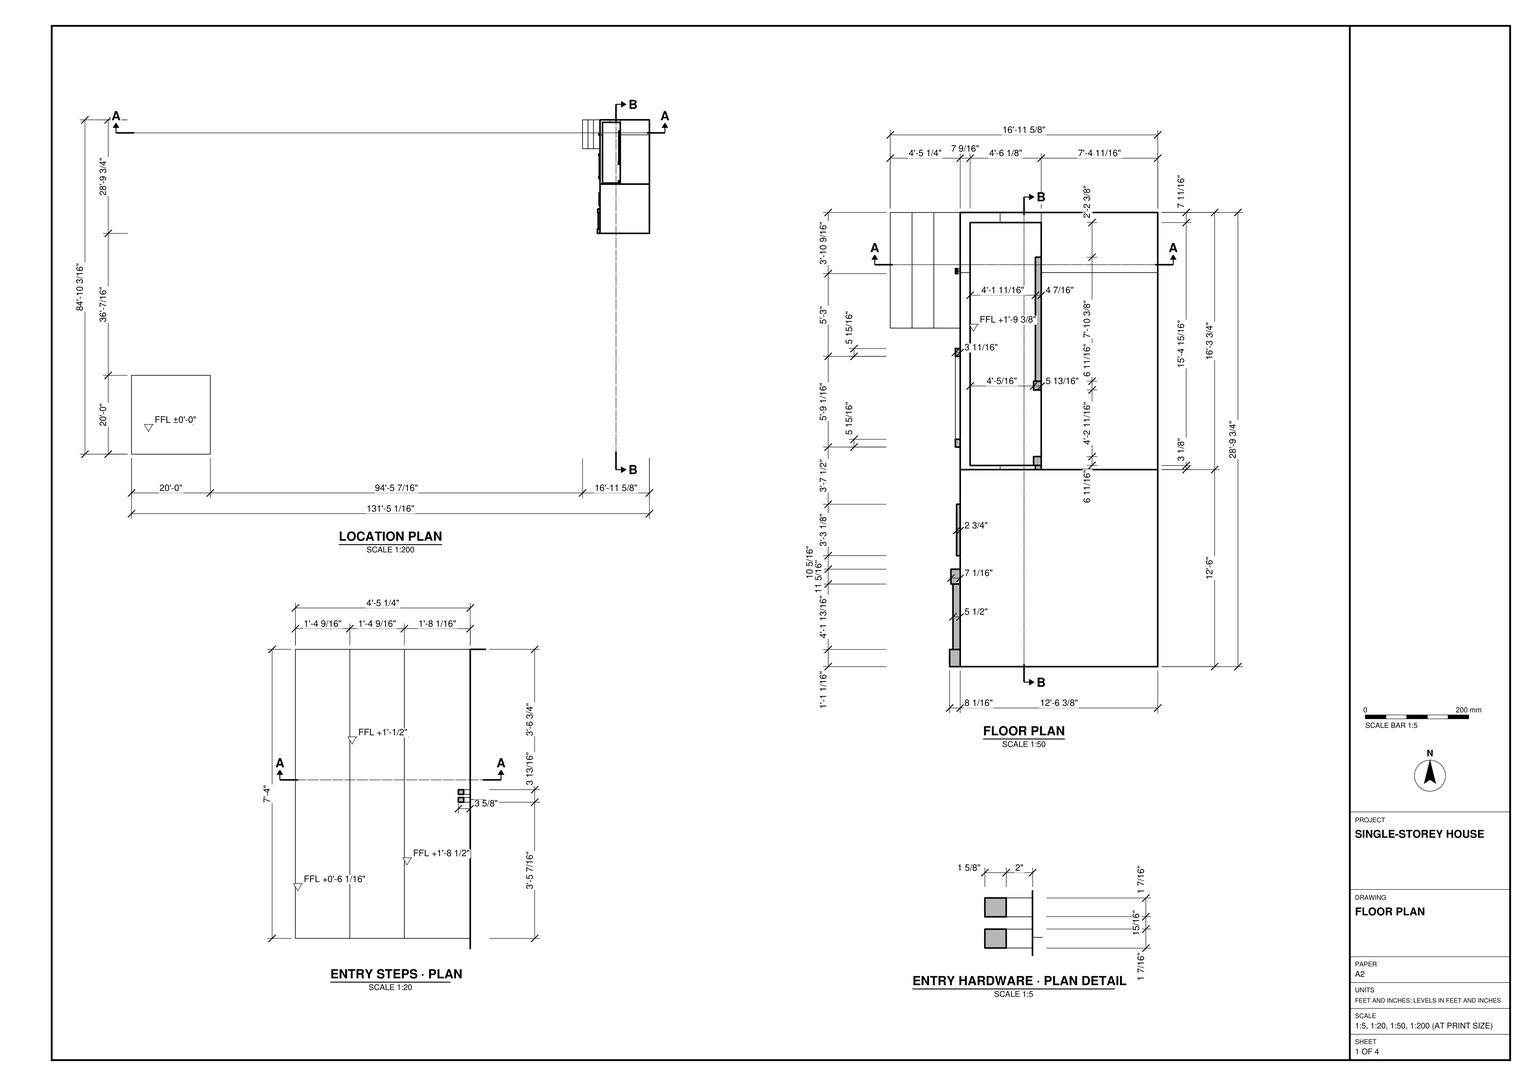
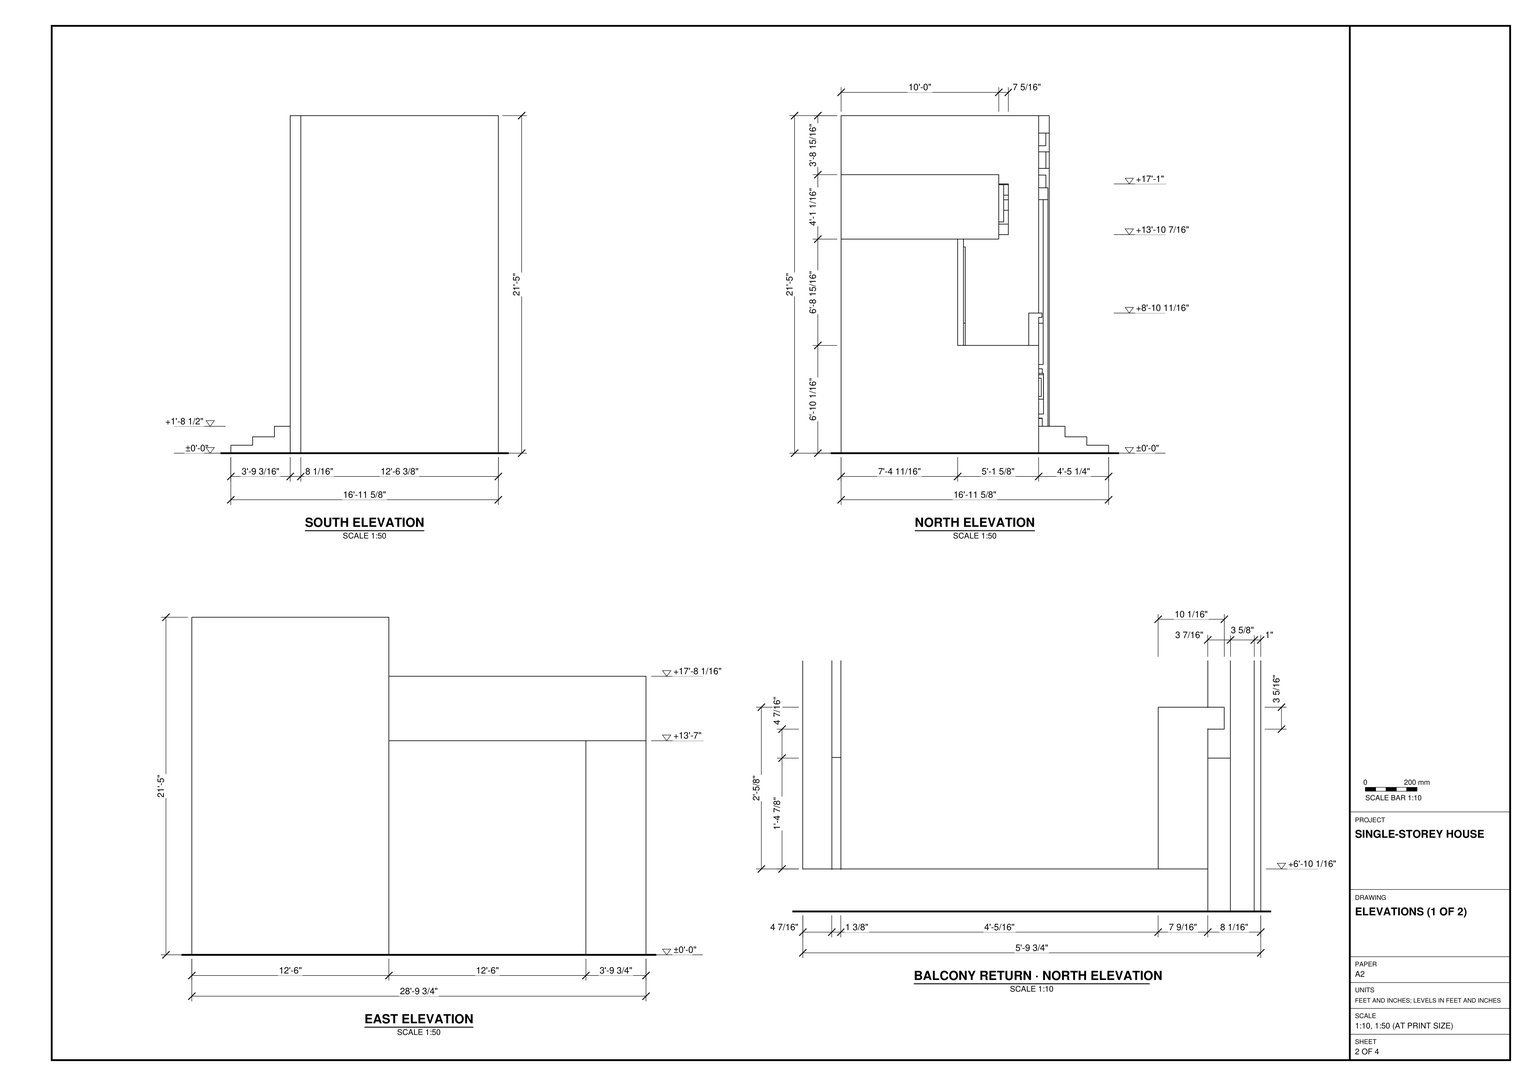
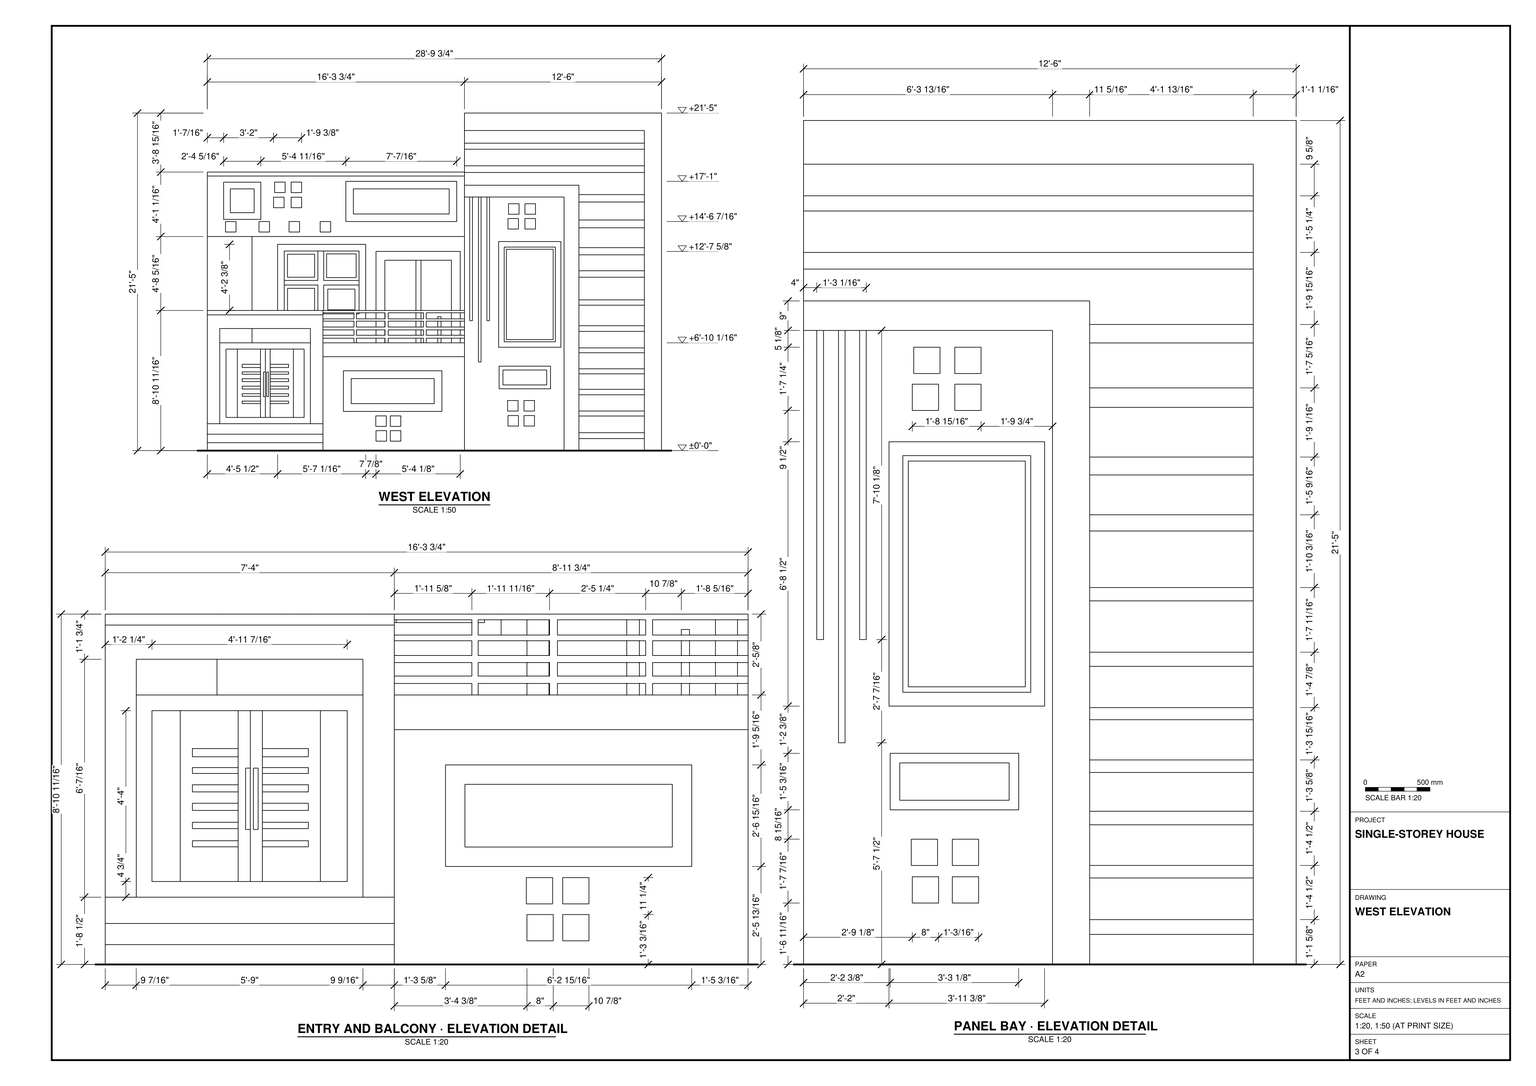
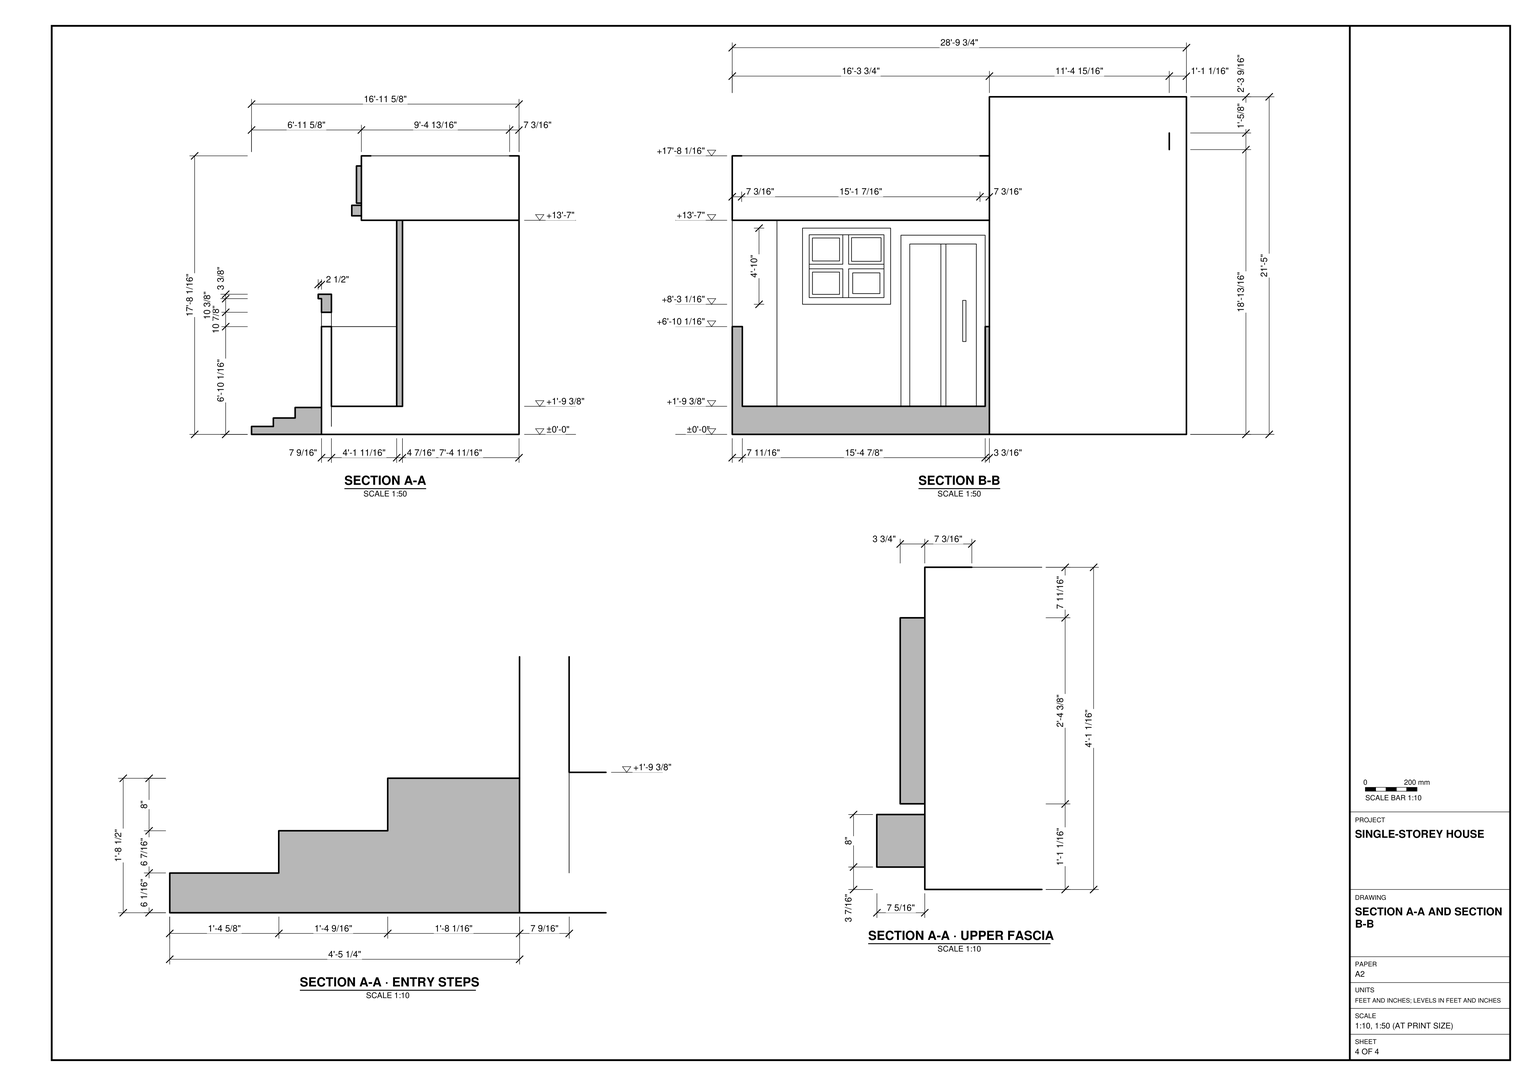
Build the house in SketchUp from task_files/diagram_01.pdf. Work in feet and inches. Use the location plan to place the separate square ground surface southwest of the house. With both in place, the overall model must measure 131'-5 1/16" along X, 84'-10 3/16" along Y and 21'-5" along Z. Use ±0'-0" as the ground-floor datum.

Form the shell with the wall thicknesses, slab edges and stepped roofline shown in the plans and elevations. Put the taller volume at the south end. On the west face, model the entry steps, paired door leaves, pulls and rectangular door surround. Beside the entrance, form the balcony with its horizontal rails, uprights and return. Use the elevation details to set out the openings, nested rectangular frames, small square features and narrow vertical strips. Distinguish the projecting panel bay from the horizontal bands behind it. Keep the other elevations as simple as drawn.

Keep walls, slabs and roof elements in separate groups or components, and group each furniture or joinery piece separately. Use components for repeated parts. Any decor or loose items shown may be suitable library components. Save one SketchUp model as output_files/single_storey_house_with_a_stepped_entrance_and_balcony.skp.

# SketchUp Ruby script. Lengths in inches.
U = 1.inch
M = Sketchup.active_model
def pt(a) = Geom::Point3d.new(a.map { |v| v * U })
def face(e, loops, mat)
  f = e.add_face(loops[0].map { |a| pt(a) })
  loops[1..].each { |l| e.add_face(l.map { |a| pt(a) }).erase! }
  f.material = f.back_material = mat if mat
  f
end
# faces: each face lists its corners as indices into pts; further lists are holes
def faces(e, pts, list, mat = nil) = list.each { |f| face(e, (f[0].is_a?(Array) ? f : [f]).map { |l| l.map { |i| pts[i] } }, mat) }
# xy, xz, yz: faces in a plane at the given z, y or x. An outline is a flat list of corners, or four numbers for a rectangle; further outlines are holes
def ring(l) = l.size == 4 ? [[l[0], l[1]], [l[2], l[1]], [l[2], l[3]], [l[0], l[3]]] : l.each_slice(2).to_a
def flat(e, list, mat, &to3) = list.each { |f| face(e, (f[0].is_a?(Array) ? f : [f]).map { |l| ring(l).map { |u, v| to3.(u, v) } }, mat) }
def xy(e, z, list, mat = nil) = flat(e, list, mat) { |x, y| [x, y, z] }
def xz(e, y, list, mat = nil) = flat(e, list, mat) { |x, z| [x, y, z] }
def yz(e, x, list, mat = nil) = flat(e, list, mat) { |y, z| [x, y, z] }
def lines(e, pts, list) = list.each { |a, b| e.add_line(pt(pts[a]), pt(pts[b])) }
# prism: a flat outline (further loops are holes) pulled along v
def prism(e, loops, v, mat = nil)
  f = face(e, loops, mat); d = Geom::Vector3d.new(v.map { |x| x * U })
  f.pushpull(f.normal.samedirection?(d) ? d.length : -d.length)
end
def box(e, o, s, mat = nil) = prism(e, [[o, [o[0] + s[0], o[1], o[2]], [o[0] + s[0], o[1] + s[1], o[2]], [o[0], o[1] + s[1], o[2]]]], [0, 0, s[2]], mat)
def at(x, y, z, deg = 0) = Geom::Transformation.translation(pt([x, y, z])) * Geom::Transformation.rotation(ORIGIN, Z_AXIS, deg.degrees)
def axes(o, x, y, z) = Geom::Transformation.new([*x, 0, *y, 0, *z, 0, *pt(o).to_a, 1])
def part(name) = M.definitions.add(name)
# library, detail: a bought-in or finely detailed component or shape, given as its bounding box
def library(name, o, s) = part(name).tap { |d| box(d.entities, o, s) }
def detail(e, o, s) = box(e.add_group.entities, o, s)
def put(e, d, t, mat = nil) = e.add_instance(d, t).tap { |i| i.material = mat if mat }
def group(e, t, mat = nil) = e.add_group.tap { |g| g.transformation = t; g.material = mat if mat }.entities
root = M.entities
M.materials.add("[0111_SlateGray]").color = [112, 128, 144]
M.materials.add("[0137_Black]").color = [0, 0, 0]
M.materials.add("[Color M00]").color = [255, 255, 255]
M.materials.add("[Color M05]").color = [114, 114, 114]
M.materials.add("[Herringbone 4x1]").color = [216, 216, 216]
M.materials.add("[Metal Seamed]").color = [118, 119, 115]
M.materials.add("[Mirror 01]").color = [185, 185, 185]
M.materials.add("[Wood Veneer 01]").color = [120, 70, 37]
xy(root,0,[[0,0,240,240],[1418.64,672.43,1426.7,685.49],[1426.7,672.43,1577.07,822.43],[1419.64,735.31,1426.7,746.62],[1426.7,822.43,1457.07,972.43],
  [1457.07,822.43,1488.375,972.43],[1488.375,822.43,1577.07,972.43],[1373.45,930.16,1426.7,972.43],[1373.45,972.43,1426.7,1018.18],[1426.7,972.43,1457.07,1018.18],
  [1457.07,972.43,1488.375,1018.18],[1488.375,972.43,1577.07,1018.18]])
xy(root,0,[[1421.2,685.49,1426.7,735.31]],"[0111_SlateGray]")
xy(root,6.05,[[1373.45,930.16,1390.04,1018.18]])
xy(root,7.2,[[1423.95,870.88,1426.7,878.88],[1423.95,881.76,1426.7,889.76]])
xy(root,9.15,[[1421.2,685.49,1426.7,735.31]],"[Color M05]")
xy(root,12.48,[[1390.04,930.16,1406.63,1018.18]])
xy(root,13.65,[[1421.2,685.49,1426.7,735.31]],"[Color M05]")
xy(root,15.2,[[1423.95,870.88,1426.7,878.88],[1423.95,881.76,1426.7,889.76]])
xy(root,18.45,[[1423.95,870.88,1426.7,878.88],[1423.95,881.94,1426.7,889.94]])
xy(root,18.7,[[1423.95,769.13,1426.7,777.13],[1423.95,781.32,1426.7,789.32]])
xy(root,20.48,[[1406.63,930.16,1426.7,1018.18]])
xy(root,21.375,[[1483.9375,822.43,1488.375,825.65],[1434.25,825.5625,1483.9375,825.65,1482.5625,825.65,1482.5625,832.36,1488.375,832.36,1488.375,883.05,1482.5625,883.05,1482.5625,889.76,1483.9375,889.76,1483.9375,984.15,1488.375,984.15,1488.375,1010.5,1434.25,1010.5],[1482.5625,825.65,1483.9375,832.36],[1483.9375,825.65,1488.375,832.36],[1482.5625,883.05,1483.9375,889.76],
  [1483.9375,883.05,1488.375,889.76],[1483.9375,889.76,1488.375,984.15]])
xy(root,26.34,[[1421.2,685.49,1426.7,735.31]],"[Color M05]")
xy(root,26.45,[[1423.95,870.88,1426.7,878.88],[1423.95,881.94,1426.7,889.94]])
xy(root,26.7,[[1423.95,769.13,1426.7,777.13],[1423.95,781.32,1426.7,789.32]])
xy(root,29.84,[[1423.01,839.59,1426.7,914.57]])
xy(root,30.14,[[1423.95,769.13,1426.7,777.13],[1423.95,781.63,1426.7,789.63]])
xy(root,30.15,[[1421.2,685.49,1426.7,735.31]],"[Color M05]")
xy(root,35.76,[[1423.01,845.5,1426.7,908.65]])
xy(root,38.14,[[1423.95,769.13,1426.7,777.13],[1423.95,781.63,1426.7,789.63]])
xy(root,41.1,[[1423.07,971.625,1426.7,973.0625],[1423.07,974,1426.7,975.4375]])
xy(root,42.52,[[1421.2,685.49,1426.7,735.31]],"[Color M05]")
xy(root,43.19,[[1424.7,971.625,1426.7,973.0625],[1424.7,974,1426.7,975.4375]])
xy(root,46.65,[[1421.2,685.49,1426.7,735.31]],"[Color M05]")
xy(root,47.08,[[1423.95,756.91,1426.7,796.06]])
xy(root,50,[[1423.95,759.83,1426.7,793.15]])
xy(root,54.86,[[1423.01,845.5,1426.7,908.65]])
xy(root,57.13,[[1424.7,971.625,1426.7,973.0625],[1424.7,974,1426.7,975.4375]])
xy(root,58.46,[[1421.2,685.49,1426.7,735.31]],"[Color M05]")
xy(root,59.79,[[1423.07,971.625,1426.7,973.0625],[1423.07,974,1426.7,975.4375]])
xy(root,60.77,[[1423.01,839.59,1426.7,914.57]])
xy(root,61.375,[[1423.95,759.83,1426.7,793.15]])
xy(root,62.27,[[1426.57,685.49,1426.7,735.31]])
xy(root,62.27,[[1421.2,685.49,1426.57,735.31]],"[Color M05]")
xy(root,64.29,[[1423.95,756.91,1426.7,796.06]])
xy(root,67.5,[[1423.26,809.79,1426.7,811.79]])
xy(root,74.52,[[1426.57,685.49,1426.7,735.31]])
xy(root,74.52,[[1421.2,685.49,1426.57,735.31]],"[Color M05]")
xy(root,78.21,[[1421.2,685.49,1426.7,735.31]],"[Color M05]")
xy(root,78.66,[[1423.95,749.04,1426.7,796.41]],"[Color M05]")
xy(root,82.0625,[[1426.7,822.43,1434.25,930.16],[1434.25,822.43,1483.9375,822.43,1483.9375,825.65,1434.25,825.5625],[1426.7,939.72,1434.25,1008.72],[1434.25,1010.5,1488.375,1018.18]])
xy(root,82.88,[[1423.95,753.25,1426.07,792.2],[1426.07,753.25,1426.7,792.2]])
xy(root,84.54,[[1426.07,754.91,1426.7,790.54]])
xy(root,90.77,[[1421.2,685.49,1426.7,735.31]],"[Color M05]")
xy(root,92.9375,[[1426.7,939.72,1434.25,1008.72]],"[Color M05]")
xy(root,95.09,[[1421.2,685.49,1426.7,735.31]],"[Color M05]")
xy(root,98.9375,[[1423.26,803.35,1426.7,805.35],[1423.26,816.35,1426.7,818.41]])
xy(root,99.04,[[1482.5625,897.62,1483.9375,964.68],[1483.9375,897.62,1488.375,964.68]])
xy(root,103.35,[[1424.2,930.16,1426.7,1018.18]],"[Color M05]")
xy(root,104.1,[[1482.5625,902.68,1483.9375,959.62],[1483.9375,902.68,1488.375,959.62]])
xy(root,106.6875,[[1424.2,930.16,1434.25,1018.18]],"[Color M05]")
xy(root,110.71,[[1421.2,685.49,1426.7,735.31]],"[Color M05]")
xy(root,114.78,[[1421.2,685.49,1426.7,735.31]],"[Color M05]")
xy(root,132,[[1421.2,685.49,1426.7,735.31]],"[Color M05]")
xy(root,136.9375,[[1421.2,685.49,1426.7,735.31]],"[Color M05]")
xy(root,144.9375,[[1482.5625,832.36,1488.375,883.05]])
xy(root,149.0625,[[1421.2,685.49,1426.7,735.31]],"[Color M05]")
xy(root,151.65,[[1482.5625,825.65,1483.9375,889.76],[1483.9375,825.65,1488.375,889.76]])
xy(root,151.97,[[1482.5625,902.68,1483.9375,959.62],[1483.9375,902.68,1488.375,959.62]])
xy(root,153.29,[[1426.07,754.91,1426.7,790.54]])
xy(root,154.51,[[1421.2,685.49,1426.7,735.31]],"[Color M05]")
xy(root,154.95,[[1426.07,753.25,1426.7,792.2]])
xy(root,154.95,[[1423.95,753.25,1426.07,792.2]],"[Color M05]")
xy(root,157.03,[[1482.5625,897.62,1483.9375,964.68],[1483.9375,897.62,1488.375,964.68]])
xy(root,159.16,[[1423.95,749.04,1426.7,796.41]],"[Color M05]")
xy(root,163,[[1457.07,822.43,1457.07,1018.18,1488.375,1018.18,1488.375,984.15,1483.9375,984.15,1483.9375,822.43],[1483.9375,822.43,1488.375,972.43],[1488.375,822.43,1577.07,1018.18],[1483.9375,972.43,1488.375,984.15]])
xy(root,166.41,[[1449.76,924.27,1457.07,932.27],[1449.76,947.96,1457.07,955.96],[1449.76,970.84,1457.07,978.84],[1449.76,996.34,1457.07,1004.34]])
xy(root,168.7,[[1423.26,768.38,1426.7,776.38],[1423.26,781.32,1426.7,789.32]])
xy(root,169.64,[[1421.2,685.49,1426.7,735.31]],"[Color M05]")
xy(root,174.41,[[1449.76,828.32,1457.07,912.74],[1449.76,924.27,1457.07,932.27],[1449.76,947.96,1457.07,955.96],[1449.76,970.84,1457.07,978.84],[1449.76,996.34,1457.07,1004.34]])
xy(root,175.57,[[1421.2,685.49,1426.7,735.31]],"[Color M05]")
xy(root,176.04,[[1453.32,977.45,1457.07,1005.77]])
xy(root,176.7,[[1423.26,768.38,1426.7,776.38],[1423.26,781.32,1426.7,789.32]])
xy(root,179.95,[[1423.26,768.38,1426.7,776.38],[1423.26,780.88,1426.7,788.88]])
xy(root,180.15,[[1449.76,834.0625,1457.07,907]])
xy(root,181.13,[[1453.32,982.54,1457.07,1000.68]])
xy(root,184.93,[[1449.76,946.38,1457.07,954.38],[1449.76,959.76,1457.07,967.76]])
xy(root,187.95,[[1423.26,768.38,1426.7,776.38],[1423.26,780.88,1426.7,788.88]])
xy(root,189.26,[[1421.2,685.49,1426.7,735.31]],"[Color M05]")
xy(root,192.93,[[1449.76,946.38,1457.07,954.38],[1449.76,959.76,1457.07,967.76]])
xy(root,193.0625,[[1419.64,746.62,1426.7,803.35],[1419.64,803.35,1423.26,805.35],[1423.26,803.35,1426.7,805.35],[1419.64,805.35,1426.7,809.79],[1419.64,809.79,1423.26,811.79],
  [1423.26,809.79,1426.7,811.79],[1419.64,811.79,1426.7,816.35],[1419.64,816.35,1423.26,818.41],[1423.26,816.35,1426.7,818.41],[1419.64,818.41,1426.7,822.43]])
xy(root,194.89,[[1421.2,685.49,1426.7,735.31]],"[Color M05]")
xy(root,196.43,[[1449.76,946.38,1457.07,954.38],[1449.76,958.95,1457.07,966.95]])
xy(root,199.27,[[1449.76,834.0625,1457.07,907],[1453.32,982.54,1457.07,1000.68]])
xy(root,202.05,[[1419.64,735.31,1421.2,822.43],[1421.2,735.31,1426.7,822.43]])
xy(root,204.36,[[1453.32,977.45,1457.07,1005.77]])
xy(root,204.43,[[1449.76,946.38,1457.07,954.38],[1449.76,958.95,1457.07,966.95]])
xy(root,205.02,[[1449.76,828.32,1457.07,912.74]])
xy(root,211.75,[[1421.2,685.49,1426.7,822.43]],"[Color M05]")
xy(root,212.0625,[[[1457.07,822.43,1577.07,1018.18],[1464.24,829.6,1569.91,1011.02]]])
xy(root,216.82,[[1421.2,685.49,1426.7,822.43]],"[Color M05]")
xy(root,229.44,[[1421.2,685.49,1426.7,822.43]],"[Color M05]")
xy(root,234.07,[[1421.26,685.49,1426.7,822.43]],"[Color M05]")
xy(root,243.69,[[1418.64,685.49,1421.26,822.43],[1421.26,685.49,1426.7,822.43]])
xy(root,257,[[1418.64,672.43,1426.7,822.43],[1426.7,672.43,1577.07,822.43]])
xz(root,672.43,[[1418.64,0,1426.7,257],[1426.7,0,1577.07,257]])
xz(root,685.49,[[1418.64,0,1418.64,216.82,1426.7,216.82,1426.7,211.75,1421.2,211.75,1421.2,194.89,1426.7,194.89,1426.7,189.26,1421.2,189.26,1421.2,175.57,1426.7,175.57,1426.7,169.64,1421.2,169.64,1421.2,154.51,1426.7,154.51,1426.7,149.0625,1421.2,149.0625,1421.2,136.9375,1426.7,136.9375,1426.7,132,1421.2,132,1421.2,114.78,1426.7,114.78,1426.7,110.71,1421.2,110.71,1421.2,95.09,1426.7,95.09,1426.7,90.77,1421.2,90.77,1421.2,78.21,1426.7,78.21,1426.7,74.52,1421.2,74.52,1421.2,62.27,1426.7,62.27,1426.7,58.46,1421.2,58.46,1421.2,46.65,1426.7,46.65,1426.7,42.52,1421.2,42.52,1421.2,30.15,1426.7,30.15,1426.7,26.34,1421.2,26.34,1421.2,13.65,1426.7,13.65,1426.7,9.15,1421.2,9.15,1421.2,0],[1421.2,0,1426.7,9.15],[1421.2,13.65,1426.7,26.34],[1421.2,30.15,1426.7,42.52],[1421.2,46.65,1426.7,58.46],
  [1421.2,62.27,1426.57,74.52],[1426.57,62.27,1426.7,74.52],[1421.2,78.21,1426.7,90.77],[1421.2,95.09,1426.7,110.71],[1421.2,114.78,1426.7,132],
  [1421.2,136.9375,1426.7,149.0625],[1421.2,154.51,1426.7,169.64],[1421.2,175.57,1426.7,189.26],[1421.2,194.89,1426.7,211.75],[1418.64,216.82,1421.2,229.44],
  [1421.2,216.82,1426.7,229.44],[1426.7,216.82,1497.89,229.44],[1418.64,229.44,1418.64,243.69,1421.26,243.69,1421.26,234.07,1426.7,234.07,1426.7,229.44],[1421.26,234.07,1426.7,243.69]])
xz(root,735.31,[[1419.64,0,1421.2,0,1421.2,9.15,1426.7,9.15,1426.7,13.65,1421.2,13.65,1421.2,26.34,1426.7,26.34,1426.7,30.15,1421.2,30.15,1421.2,42.52,1426.7,42.52,1426.7,46.65,1421.2,46.65,1421.2,58.46,1426.7,58.46,1426.7,62.27,1421.2,62.27,1421.2,74.52,1426.7,74.52,1426.7,78.21,1421.2,78.21,1421.2,90.77,1426.7,90.77,1426.7,95.09,1421.2,95.09,1421.2,110.71,1426.7,110.71,1426.7,114.78,1421.2,114.78,1421.2,132,1426.7,132,1426.7,136.9375,1421.2,136.9375,1421.2,149.0625,1426.7,149.0625,1426.7,154.51,1421.2,154.51,1421.2,169.64,1426.7,169.64,1426.7,175.57,1421.2,175.57,1421.2,189.26,1426.7,189.26,1426.7,194.89,1421.2,194.89,1421.2,202.05,1419.64,202.05],[1421.2,0,1426.7,9.15],[1421.2,13.65,1426.7,26.34],[1421.2,30.15,1426.7,42.52],[1421.2,46.65,1426.7,58.46],
  [1421.2,62.27,1426.57,74.52],[1426.57,62.27,1426.7,74.52],[1421.2,78.21,1426.7,90.77],[1421.2,95.09,1426.7,110.71],[1421.2,114.78,1426.7,132],
  [1421.2,136.9375,1426.7,149.0625],[1421.2,154.51,1426.7,169.64],[1421.2,175.57,1426.7,189.26],[1421.2,194.89,1426.7,202.05]])
xz(root,746.62,[[1419.64,0,1426.7,193.0625]])
xz(root,749.04,[[1423.95,78.66,1426.7,159.16]],"[Color M05]")
xz(root,753.25,[[1426.07,82.88,1426.7,154.95]])
xz(root,753.25,[[1423.95,82.88,1426.07,154.95]],"[Color M05]")
xz(root,754.91,[[1426.07,84.54,1426.7,153.29]])
xz(root,756.91,[[1423.95,47.08,1426.7,64.29]])
xz(root,759.83,[[1423.95,50,1426.7,61.375]])
xz(root,768.38,[[1423.26,168.7,1426.7,176.7],[1423.26,179.95,1426.7,187.95]])
xz(root,769.13,[[1423.95,18.7,1426.7,26.7],[1423.95,30.14,1426.7,38.14]])
xz(root,776.38,[[1423.26,168.7,1426.7,176.7],[1423.26,179.95,1426.7,187.95]])
xz(root,777.13,[[1423.95,18.7,1426.7,26.7],[1423.95,30.14,1426.7,38.14]])
xz(root,780.88,[[1423.26,179.95,1426.7,187.95]])
xz(root,781.32,[[1423.95,18.7,1426.7,26.7],[1423.26,168.7,1426.7,176.7]])
xz(root,781.63,[[1423.95,30.14,1426.7,38.14]])
xz(root,788.88,[[1423.26,179.95,1426.7,187.95]])
xz(root,789.32,[[1423.95,18.7,1426.7,26.7],[1423.26,168.7,1426.7,176.7]])
xz(root,789.63,[[1423.95,30.14,1426.7,38.14]])
xz(root,790.54,[[1426.07,84.54,1426.7,153.29]])
xz(root,792.2,[[1426.07,82.88,1426.7,154.95]])
xz(root,792.2,[[1423.95,82.88,1426.07,154.95]],"[0111_SlateGray]")
xz(root,793.15,[[1423.95,50,1426.7,61.375]])
xz(root,796.06,[[1423.95,47.08,1426.7,64.29]],"[Color M00]")
xz(root,796.41,[[1423.95,78.66,1426.7,159.16]],"[Color M05]")
xz(root,803.35,[[1423.26,98.9375,1426.7,193.0625]])
xz(root,805.35,[[1423.26,98.9375,1426.7,193.0625]])
xz(root,809.79,[[1423.26,67.5,1426.7,193.0625]])
xz(root,811.79,[[1423.26,67.5,1426.7,193.0625]])
xz(root,816.35,[[1423.26,98.9375,1426.7,193.0625]])
xz(root,818.41,[[1423.26,98.9375,1426.7,193.0625]])
xz(root,822.43,[[1426.7,0,1457.07,82.0625],[1457.07,0,1488.375,21.375],[1488.375,0,1577.07,163],[1457.07,21.375,1483.9375,82.0625],[1483.9375,21.375,1488.375,163],
  [1426.7,82.0625,1426.7,257,1577.07,257,1577.07,212.0625,1457.07,212.0625,1457.07,163,1483.9375,163,1483.9375,82.0625],[1457.07,163,1577.07,212.0625],[1419.64,193.0625,1426.7,202.05],[1418.64,243.69,1426.7,257]])
xz(root,822.43,[[1421.2,202.05,1426.7,211.75],[1421.2,216.82,1426.7,229.44],[1421.26,234.07,1426.7,243.69]],"[0111_SlateGray]")
xz(root,825.65,[[1482.5625,21.375,1483.9375,151.65],[1483.9375,21.375,1488.375,151.65]])
xz(root,828.32,[[1449.76,174.41,1457.07,205.02]])
xz(root,832.36,[[1482.5625,21.375,1488.375,144.9375]])
xz(root,834.0625,[[1449.76,180.15,1457.07,199.27]])
xz(root,839.59,[[1423.01,29.84,1426.7,60.77]])
xz(root,845.5,[[1423.01,35.76,1426.7,54.86]])
xz(root,870.88,[[1423.95,7.2,1426.7,15.2],[1423.95,18.45,1426.7,26.45]])
xz(root,878.88,[[1423.95,7.2,1426.7,15.2],[1423.95,18.45,1426.7,26.45]])
xz(root,881.76,[[1423.95,7.2,1426.7,15.2]])
xz(root,881.94,[[1423.95,18.45,1426.7,26.45]])
xz(root,883.05,[[1482.5625,21.375,1488.375,144.9375]])
xz(root,889.76,[[1423.95,7.2,1426.7,15.2],[1482.5625,21.375,1483.9375,151.65],[1483.9375,21.375,1488.375,151.65]])
xz(root,889.94,[[1423.95,18.45,1426.7,26.45]])
xz(root,897.62,[[1482.5625,99.04,1483.9375,157.03],[1483.9375,99.04,1488.375,157.03]])
xz(root,902.68,[[1482.5625,104.1,1483.9375,151.97],[1483.9375,104.1,1488.375,151.97]])
xz(root,907,[[1449.76,180.15,1457.07,199.27]])
xz(root,908.65,[[1423.01,35.76,1426.7,54.86]])
xz(root,912.74,[[1449.76,174.41,1457.07,205.02]])
xz(root,914.57,[[1423.01,29.84,1426.7,60.77]])
xz(root,924.27,[[1449.76,166.41,1457.07,174.41]])
xz(root,930.16,[[1373.45,0,1426.7,0,1426.7,20.48,1406.63,20.48,1406.63,12.48,1390.04,12.48,1390.04,6.05,1373.45,6.05]])
xz(root,930.16,[[1426.7,82.0625,1434.25,82.0625,1434.25,106.6875,1424.2,106.6875,1424.2,103.35,1426.7,103.35]],"[Color M05]")
xz(root,932.27,[[1449.76,166.41,1457.07,174.41]])
xz(root,939.72,[[1426.7,82.0625,1434.25,92.9375]],"[Color M05]")
xz(root,946.38,[[1449.76,184.93,1457.07,192.93],[1449.76,196.43,1457.07,204.43]])
xz(root,947.96,[[1449.76,166.41,1457.07,174.41]])
xz(root,954.38,[[1449.76,184.93,1457.07,192.93],[1449.76,196.43,1457.07,204.43]])
xz(root,955.96,[[1449.76,166.41,1457.07,174.41]])
xz(root,958.95,[[1449.76,196.43,1457.07,204.43]])
xz(root,959.62,[[1482.5625,104.1,1483.9375,151.97],[1483.9375,104.1,1488.375,151.97]])
xz(root,959.76,[[1449.76,184.93,1457.07,192.93]])
xz(root,964.68,[[1482.5625,99.04,1483.9375,157.03],[1483.9375,99.04,1488.375,157.03]])
xz(root,966.95,[[1449.76,196.43,1457.07,204.43]])
xz(root,967.76,[[1449.76,184.93,1457.07,192.93]])
xz(root,970.84,[[1449.76,166.41,1457.07,174.41]])
xz(root,971.625,[[1423.07,41.1,1426.7,41.1,1426.7,43.19,1424.7,43.19,1424.7,57.13,1426.7,57.13,1426.7,59.79,1423.07,59.79]])
xz(root,973.0625,[[1423.07,41.1,1423.07,59.79,1426.7,59.79,1426.7,57.13,1424.7,57.13,1424.7,43.19,1426.7,43.19,1426.7,41.1]])
xz(root,974,[[1423.07,41.1,1426.7,41.1,1426.7,43.19,1424.7,43.19,1424.7,57.13,1426.7,57.13,1426.7,59.79,1423.07,59.79]])
xz(root,975.4375,[[1423.07,41.1,1423.07,59.79,1426.7,59.79,1426.7,57.13,1424.7,57.13,1424.7,43.19,1426.7,43.19,1426.7,41.1]])
xz(root,977.45,[[1453.32,176.04,1457.07,204.36]])
xz(root,978.84,[[1449.76,166.41,1457.07,174.41]])
xz(root,982.54,[[1453.32,181.13,1457.07,199.27]])
xz(root,984.15,[[1483.9375,21.375,1488.375,163]])
xz(root,996.34,[[1449.76,166.41,1457.07,174.41]])
xz(root,1000.68,[[1453.32,181.13,1457.07,199.27]])
xz(root,1004.34,[[1449.76,166.41,1457.07,174.41]])
xz(root,1005.77,[[1453.32,176.04,1457.07,204.36]])
xz(root,1008.72,[[1426.7,82.0625,1434.25,92.9375]],"[Color M05]")
xz(root,1010.5,[[1434.25,21.375,1488.375,82.0625]])
xz(root,1018.18,[[1373.45,0,1373.45,6.05,1390.04,6.05,1390.04,12.48,1406.63,12.48,1406.63,20.48,1426.7,20.48,1426.7,0],[1426.7,0,1426.7,82.0625,1488.375,82.0625,1488.375,163,1577.07,163,1577.07,0],[1457.07,163,1577.07,212.0625]])
xz(root,1018.18,[[1426.7,82.0625,1426.7,103.35,1424.2,103.35,1424.2,106.6875,1434.25,106.6875,1434.25,82.0625]],"[Color M05]")
yz(root,1373.45,[[930.16,0,1018.18,6.05]])
yz(root,1390.04,[[930.16,6.05,1018.18,12.48]])
yz(root,1406.63,[[930.16,12.48,1018.18,20.48]])
yz(root,1418.64,[[672.43,0,672.43,257,822.43,257,822.43,243.69,685.49,243.69,685.49,0]],"[Color M00]")
yz(root,1419.64,[[735.31,0,735.31,202.05,822.43,202.05,822.43,193.0625,746.62,193.0625,746.62,0]],"[Color M00]")
yz(root,1421.2,[[685.49,0,735.31,9.15],[685.49,13.65,735.31,26.34],[685.49,30.15,735.31,42.52],[685.49,46.65,735.31,58.46],[685.49,62.27,735.31,74.52],
  [685.49,78.21,735.31,90.77],[685.49,95.09,735.31,110.71],[685.49,114.78,735.31,132],[685.49,136.9375,735.31,149.0625],[685.49,154.51,735.31,169.64],
  [685.49,175.57,735.31,189.26],[685.49,194.89,685.49,211.75,822.43,211.75,822.43,202.05,735.31,202.05,735.31,194.89],[685.49,216.82,822.43,229.44]],"[Color M05]")
yz(root,1421.26,[[685.49,234.07,822.43,243.69]],"[Color M05]")
yz(root,1423.01,[[[839.59,29.84,914.57,60.77],[845.5,35.76,908.65,54.86]]],"[Color M00]")
yz(root,1423.07,[[971.625,41.1,973.0625,59.79],[974,41.1,975.4375,59.79]])
yz(root,1423.26,[[809.79,67.5,811.79,193.0625],[803.35,98.9375,805.35,193.0625],[816.35,98.9375,818.41,193.0625],[768.38,168.7,776.38,176.7],[781.32,168.7,789.32,176.7],
  [768.38,179.95,776.38,187.95],[780.88,179.95,788.88,187.95]])
yz(root,1423.95,[[870.88,7.2,878.88,15.2],[881.76,7.2,889.76,15.2],[870.88,18.45,878.88,26.45],[881.94,18.45,889.94,26.45],[769.13,18.7,777.13,26.7],
  [781.32,18.7,789.32,26.7],[769.13,30.14,777.13,38.14],[781.63,30.14,789.63,38.14]])
yz(root,1423.95,[[[756.91,47.08,796.06,64.29],[759.83,50,793.15,61.375]]],"[Color M00]")
yz(root,1423.95,[[[749.04,78.66,796.41,159.16],[753.25,82.88,792.2,154.95]]],"[Color M05]")
yz(root,1424.2,[[930.16,103.35,1018.18,106.6875]],"[Color M05]")
yz(root,1424.7,[[971.625,43.19,973.0625,57.13],[974,43.19,975.4375,57.13]])
yz(root,1426.07,[[[753.25,82.88,792.2,154.95],[754.91,84.54,790.54,153.29]]])
yz(root,1426.57,[[685.49,62.27,735.31,74.52]])
yz(root,1426.7,[[672.43,0,685.49,0,685.49,243.69,822.43,243.69,822.43,257,672.43,257],[685.49,0,735.31,9.15],[735.31,0,746.62,0,746.62,193.0625,822.43,193.0625,822.43,202.05,735.31,202.05],[[822.43,0,930.16,71.51],[839.59,29.84,914.57,60.77],[881.94,18.45,889.94,26.45],[870.88,18.45,878.88,26.45],[870.88,7.2,878.88,15.2],[881.76,7.2,889.76,15.2]],[930.16,0,1018.18,20.48],
  [870.88,7.2,878.88,15.2],[881.76,7.2,889.76,15.2],[685.49,9.15,735.31,13.65],[685.49,13.65,735.31,26.34],[870.88,18.45,878.88,26.45],
  [881.94,18.45,889.94,26.45],[769.13,18.7,777.13,26.7],[781.32,18.7,789.32,26.7],[944.49,25.26,952.66,77.29],[995.34,25.26,1003.95,77.29],
  [685.49,26.34,735.31,30.15],[[839.59,29.84,914.57,60.77],[845.5,35.76,908.65,54.86]],[769.13,30.14,777.13,38.14],[781.63,30.14,789.63,38.14],[685.49,30.15,735.31,42.52],
  [956.33,35.82,970.33,37.67],[977.71,35.82,991.63,37.67],[971.625,41.1,973.0625,43.19],[974,41.1,975.4375,43.19],[956.33,41.37,970.33,43.3],
  [977.71,41.37,991.63,43.3],[685.49,42.52,735.31,46.65],[685.49,46.65,735.31,58.46],[956.33,46.9,970.33,49.09],[977.71,46.9,991.63,49.09],
  [[756.91,47.08,796.06,64.29],[759.83,50,793.15,61.375]],[956.33,52.55,970.33,54.72],[977.71,52.55,991.63,54.72],[971.625,57.13,973.0625,59.79],[974,57.13,975.4375,59.79],
  [956.33,58.16,970.33,59.94],[977.71,58.16,991.63,59.94],[685.49,58.46,735.31,62.27],[685.49,62.27,735.31,74.52],[956.33,63.25,970.33,65.74],
  [977.71,63.25,991.63,65.74],[809.79,67.5,811.79,193.0625],[822.43,71.51,930.16,82.0625],[685.49,74.52,735.31,78.21],[685.49,78.21,735.31,90.77],
  [[749.04,78.66,796.41,159.16],[753.25,82.88,792.2,154.95]],[[753.25,82.88,792.2,154.95],[754.91,84.54,790.54,153.29]],[685.49,90.77,735.31,95.09],[685.49,95.09,735.31,110.71],[803.35,98.9375,805.35,193.0625],
  [816.35,98.9375,818.41,193.0625],[685.49,110.71,735.31,114.78],[685.49,114.78,735.31,132],[685.49,132,735.31,136.9375],[685.49,136.9375,735.31,149.0625],
  [685.49,149.0625,735.31,154.51],[685.49,154.51,735.31,169.64],[768.38,168.7,776.38,176.7],[781.32,168.7,789.32,176.7],[685.49,169.64,735.31,175.57],
  [685.49,175.57,735.31,189.26],[768.38,179.95,776.38,187.95],[780.88,179.95,788.88,187.95],[685.49,194.89,735.31,194.89,735.31,202.05,822.43,202.05,822.43,211.75,685.49,211.75],[685.49,216.82,822.43,229.44],
  [685.49,234.07,822.43,243.69]])
yz(root,1426.7,[[[939.72,20.48,1008.72,82.0625],[944.49,25.26,1003.95,77.29]],[952.66,25.26,952.66,77.29,970.33,77.29,970.33,65.74,956.33,65.74,956.33,63.25,970.33,63.25,970.33,59.94,956.33,59.94,956.33,58.16,970.33,58.16,970.33,54.72,956.33,54.72,956.33,52.55,970.33,52.55,970.33,49.09,956.33,49.09,956.33,46.9,970.33,46.9,970.33,43.3,956.33,43.3,956.33,41.37,970.33,41.37,970.33,37.67,956.33,37.67,956.33,35.82,970.33,35.82,970.33,25.26],[[970.33,25.26,974,77.29],[971.625,57.13,973.0625,59.79],[971.625,41.1,973.0625,43.19]],[974,25.26,974,41.1,975.4375,41.1,975.4375,43.19,974,43.19,974,57.13,975.4375,57.13,975.4375,59.79,974,59.79,974,77.29,977.71,77.29,977.71,25.26],[977.71,25.26,977.71,35.82,991.63,35.82,991.63,37.67,977.71,37.67,977.71,41.37,991.63,41.37,991.63,43.3,977.71,43.3,977.71,46.9,991.63,46.9,991.63,49.09,977.71,49.09,977.71,52.55,991.63,52.55,991.63,54.72,977.71,54.72,977.71,58.16,991.63,58.16,991.63,59.94,977.71,59.94,977.71,63.25,991.63,63.25,991.63,65.74,977.71,65.74,977.71,77.29,995.34,77.29,995.34,25.26]],"[0137_Black]")
yz(root,1426.7,[[[746.62,0,746.62,193.0625,803.35,193.0625,803.35,98.9375,805.35,98.9375,805.35,193.0625,809.79,193.0625,809.79,67.5,811.79,67.5,811.79,193.0625,816.35,193.0625,816.35,98.9375,818.41,98.9375,818.41,193.0625,822.43,193.0625,822.43,0],[749.04,78.66,796.41,159.16],[756.91,47.08,796.06,64.29],[780.88,179.95,788.88,187.95],[768.38,179.95,776.38,187.95],[768.38,168.7,776.38,176.7],[781.32,168.7,789.32,176.7],[781.32,18.7,789.32,26.7],[769.13,18.7,777.13,26.7],[769.13,30.14,777.13,38.14],[781.63,30.14,789.63,38.14]],[685.49,189.26,735.31,194.89],[685.49,211.75,822.43,216.82],[685.49,229.44,822.43,234.07]],"[Color M00]")
yz(root,1426.7,[[930.16,20.48,930.16,103.35,1018.18,103.35,1018.18,20.48,1008.72,20.48,1008.72,92.9375,939.72,92.9375,939.72,20.48],[845.5,35.76,908.65,54.86],[759.83,50,793.15,61.375]],"[Color M05]")
yz(root,1426.7,[[754.91,84.54,790.54,153.29]],"[Herringbone 4x1]")
yz(root,1434.25,[[825.5625,21.375,939.72,82.0625],[939.72,21.375,1008.72,82.0625],[1008.72,21.375,1010.5,82.0625],[930.16,82.0625,939.72,92.9375],[1008.72,82.0625,1010.5,92.9375],
  [1010.5,82.0625,1018.18,92.9375],[930.16,92.9375,939.72,100.3125],[939.72,92.9375,1008.72,100.3125],[1008.72,92.9375,1010.5,100.3125],[1010.5,92.9375,1018.18,100.3125],
  [930.16,100.3125,939.72,106.6875],[939.72,100.3125,1008.72,106.6875],[1008.72,100.3125,1010.5,106.6875],[1010.5,100.3125,1018.18,106.6875]])
yz(root,1434.25,[[[851.5,82.0625,853.61,82.0625,853.61,85.57,880.48,85.57,880.48,82.0625,882.88,82.0625,882.88,85.57,904.62,85.57,904.62,82.0625,906.54,82.0625,906.54,85.57,930.16,85.57,930.16,87.82,906.54,87.82,906.54,91.93,930.16,91.93,930.16,94.09,906.54,94.09,906.54,98.58,930.16,98.58,930.16,100.3125,906.54,100.3125,906.54,104.96,930.16,104.96,930.16,106.6875,822.43,106.6875,822.43,104.96,851.5,104.96,851.5,100.3125,822.43,100.3125,822.43,98.58,851.5,98.58,851.5,94.09,822.43,94.09,822.43,91.93,851.5,91.93,851.5,87.82,822.43,87.82,822.43,85.57,851.5,85.57],[853.61,100.3125,880.48,104.96],[853.61,94.09,880.48,98.58],[853.61,87.82,880.48,91.93],[882.88,100.3125,904.62,104.96],[882.88,94.09,904.62,98.58],[882.88,87.82,904.62,91.93]]],"[Metal Seamed]")
yz(root,1449.76,[[924.27,166.41,932.27,174.41],[947.96,166.41,955.96,174.41],[970.84,166.41,978.84,174.41],[996.34,166.41,1004.34,174.41],[[828.32,174.41,912.74,205.02],[834.0625,180.15,907,199.27]],
  [946.38,184.93,954.38,192.93],[959.76,184.93,967.76,192.93],[946.38,196.43,954.38,204.43],[958.95,196.43,966.95,204.43]])
yz(root,1453.32,[[[977.45,176.04,1005.77,204.36],[982.54,181.13,1000.68,199.27]]])
yz(root,1457.07,[[924.27,166.41,932.27,174.41],[947.96,166.41,955.96,174.41],[970.84,166.41,978.84,174.41],[996.34,166.41,1004.34,174.41],[[828.32,174.41,912.74,205.02],[834.0625,180.15,907,199.27]],
  [[977.45,176.04,1005.77,204.36],[982.54,181.13,1000.68,199.27]],[946.38,184.93,954.38,192.93],[959.76,184.93,967.76,192.93],[946.38,196.43,954.38,204.43],[958.95,196.43,966.95,204.43],
  [822.43,209.04,1018.18,212.0625]])
yz(root,1457.07,[[[822.43,163,1018.18,209.04],[828.32,174.41,912.74,205.02],[977.45,176.04,1005.77,204.36],[958.95,196.43,966.95,204.43],[946.38,196.43,954.38,204.43],[946.38,184.93,954.38,192.93],[959.76,184.93,967.76,192.93],[996.34,166.41,1004.34,174.41],[970.84,166.41,978.84,174.41],[947.96,166.41,955.96,174.41],[924.27,166.41,932.27,174.41]],[834.0625,180.15,907,199.27],[982.54,181.13,1000.68,199.27]],"[Color M05]")
yz(root,1482.5625,[[825.65,21.375,825.65,151.65,889.76,151.65,889.76,21.375,883.05,21.375,883.05,144.9375,832.36,144.9375,832.36,21.375],[[897.62,99.04,964.68,157.03],[902.68,104.1,959.62,151.97]]])
yz(root,1483.9375,[[822.43,21.375,825.65,82.0625],[[889.76,21.375,889.76,151.65,825.65,151.65,825.65,82.0625,822.43,82.0625,822.43,163,984.15,163,984.15,21.375],[897.62,99.04,964.68,157.03]],[[897.62,99.04,964.68,157.03],[902.68,104.1,959.62,151.97]]])
yz(root,1488.375,[[825.65,14.66,889.76,21.375],[[822.43,21.375,825.65,21.375,825.65,151.65,889.76,151.65,889.76,21.375,984.15,21.375,984.15,163,822.43,163],[897.62,99.04,964.68,157.03]],[825.65,21.375,832.36,21.375,832.36,144.9375,883.05,144.9375,883.05,21.375,889.76,21.375,889.76,151.65,825.65,151.65],[855.53,21.375,859.37,144.9375],[840.26,70.69,842.76,102]])
yz(root,1488.375,[[984.15,21.375,984.15,163,1018.18,163,1018.18,82.0625,1010.5,82.0625,1010.5,21.375]],"[Color M05]")
yz(root,1488.375,[[936.53,106.6,957.12,123.5625],[905.78,107.2,926.49,122.96],[904.89,131.75,927.38,149.76],[936.5,132,957.15,149.51]],"[Mirror 01]")
yz(root,1488.375,[[[832.36,21.375,855.53,144.9375],[840.26,70.69,842.76,102]],[859.37,21.375,883.05,144.9375],[929.59,104.1,929.59,126.06,902.68,126.06,902.68,129.54,929.59,129.54,929.59,151.97,934.03,151.97,934.03,129.54,959.62,129.54,959.62,126.06,934.03,126.06,934.03,104.1],[[902.68,104.1,929.59,126.06],[905.78,107.2,926.49,122.96]],[[934.03,104.1,959.62,126.06],[936.53,106.6,957.12,123.5625]],
  [[902.68,129.54,929.59,151.97],[904.89,131.75,927.38,149.76]],[[934.03,129.54,959.62,151.97],[936.5,132,957.15,149.51]]],"[Wood Veneer 01]")
yz(root,1577.07,[[672.43,0,822.43,257],[822.43,0,972.43,163],[972.43,0,1018.18,163],[822.43,163,1018.18,212.0625]])
p = [[1483.9375,825.65,21.375],[1434.25,825.5625,21.375],[1434.25,825.5625,82.0625],[1483.9375,825.65,82.0625],[1488.375,1018.18,21.375],[1488.375,1010.5,21.375],
  [1434.25,822.43,104.96],[1434.25,822.43,100.3125],[1434.25,822.43,98.58],[1434.25,822.43,94.09],[1434.25,822.43,91.93],[1434.25,822.43,87.82],
  [1434.25,822.43,85.57],[1434.25,822.43,82.0625],[1434.25,1008.72,21.375],[1434.25,1008.72,6.0625]]
faces(root,p,[[0,1,2,3]])
lines(root,p,[[4,5],[6,7],[8,9],[10,11],[12,13],[14,15]])
